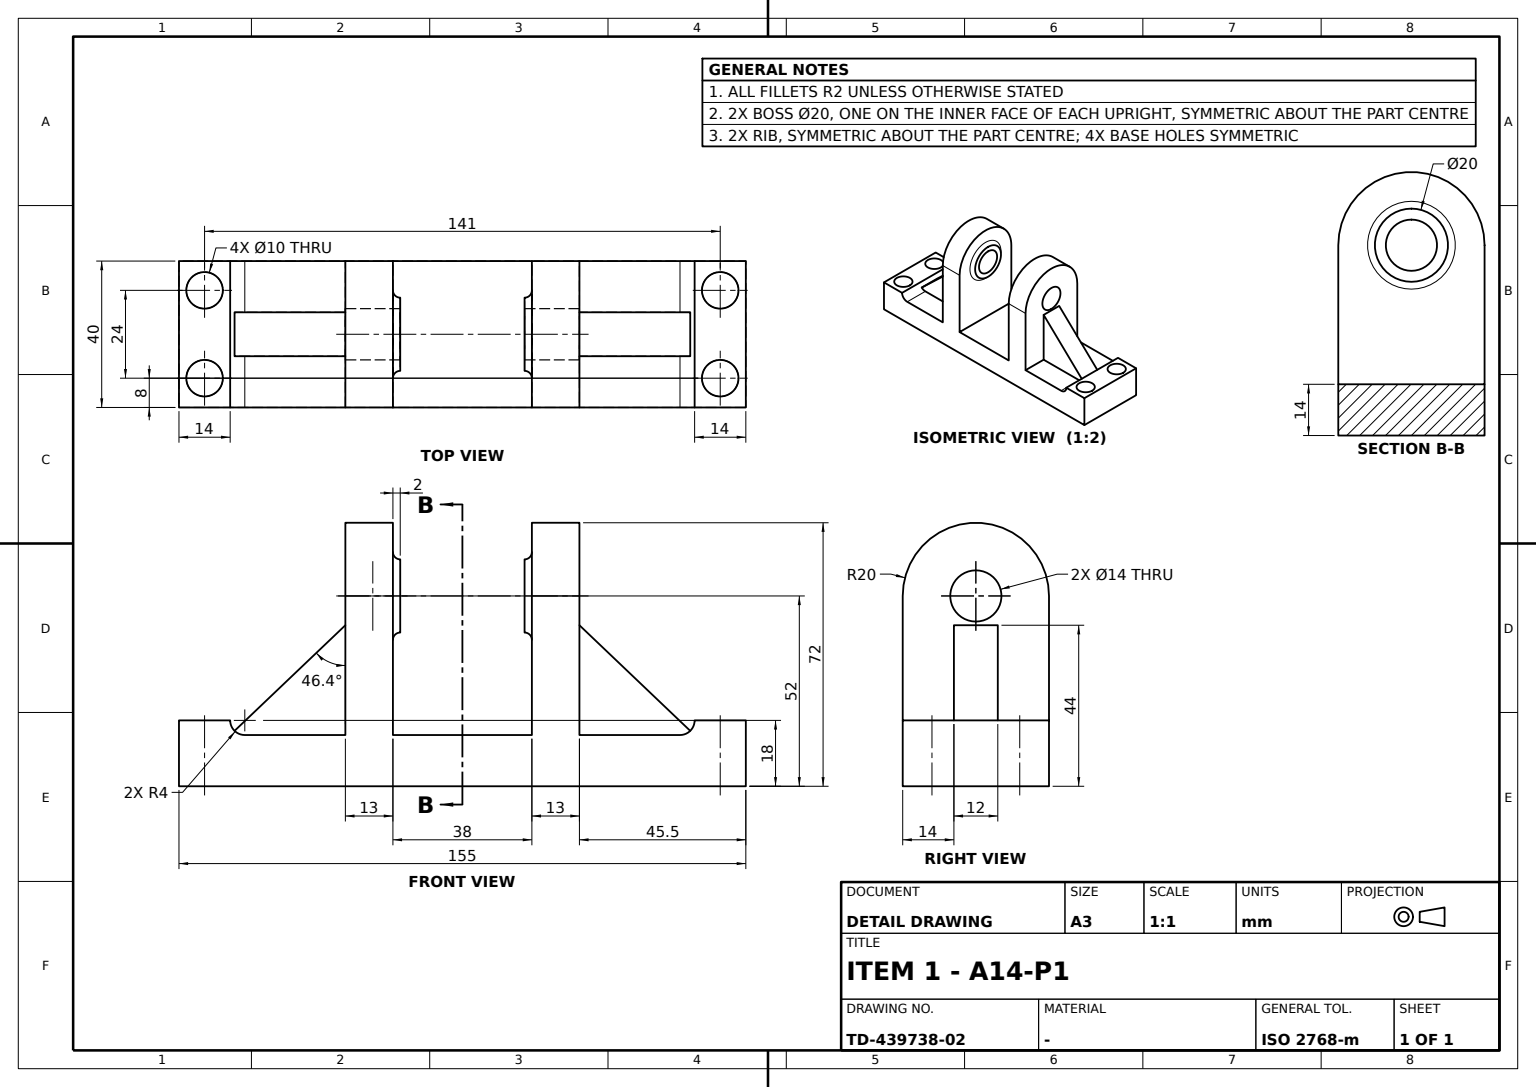
ISO-10303-21;
HEADER;
FILE_DESCRIPTION((''),'2;1');
FILE_NAME('','',(''),(''),'','','');
FILE_SCHEMA(('AUTOMOTIVE_DESIGN'));
ENDSEC;
DATA;
#1=APPLICATION_CONTEXT('');
#2=PRODUCT_CONTEXT('',#1,'mechanical');
#3=PRODUCT('','','',(#2));
#4=PRODUCT_DEFINITION_FORMATION('','',#3);
#5=PRODUCT_DEFINITION_CONTEXT('',#1,'design');
#6=PRODUCT_DEFINITION('','',#4,#5);
#7=PRODUCT_DEFINITION_SHAPE('','',#6);
#8=(LENGTH_UNIT()NAMED_UNIT(*)SI_UNIT(.MILLI.,.METRE.));
#9=(NAMED_UNIT(*)PLANE_ANGLE_UNIT()SI_UNIT($,.RADIAN.));
#10=(NAMED_UNIT(*)SI_UNIT($,.STERADIAN.)SOLID_ANGLE_UNIT());
#11=UNCERTAINTY_MEASURE_WITH_UNIT(LENGTH_MEASURE(0.005),#8,'distance_accuracy_value','');
#12=(GEOMETRIC_REPRESENTATION_CONTEXT(3)GLOBAL_UNCERTAINTY_ASSIGNED_CONTEXT((#11))GLOBAL_UNIT_ASSIGNED_CONTEXT((#8,#9,#10))REPRESENTATION_CONTEXT('',''));
#13=CARTESIAN_POINT('',(17.,0.,42.));
#14=VERTEX_POINT('',#13);
#15=CARTESIAN_POINT('',(17.,0.,52.));
#16=DIRECTION('',(1.,0.,0.));
#17=DIRECTION('',(0.,0.,-1.));
#18=AXIS2_PLACEMENT_3D('',#15,#16,#17);
#19=CIRCLE('',#18,10.);
#20=EDGE_CURVE('',#14,#14,#19,.T.);
#21=ORIENTED_EDGE('',*,*,#20,.F.);
#22=EDGE_LOOP('',(#21));
#23=FACE_BOUND('',#22,.T.);
#24=CARTESIAN_POINT('',(17.,0.,45.));
#25=VERTEX_POINT('',#24);
#26=CIRCLE('',#18,7.);
#27=EDGE_CURVE('',#25,#25,#26,.T.);
#28=ORIENTED_EDGE('',*,*,#27,.T.);
#29=EDGE_LOOP('',(#28));
#30=FACE_BOUND('',#29,.T.);
#31=CARTESIAN_POINT('',(17.,0.,14.));
#32=DIRECTION('',(0.,0.,1.));
#33=AXIS2_PLACEMENT_3D('',#31,#16,#32);
#34=PLANE('',#33);
#35=ADVANCED_FACE('',(#23,#30),#34,.F.);
#36=CARTESIAN_POINT('',(-75.5,12.,0.));
#37=VERTEX_POINT('',#36);
#38=CARTESIAN_POINT('',(-70.5,12.,0.));
#39=DIRECTION('',(-1.,0.,0.));
#40=AXIS2_PLACEMENT_3D('',#38,#17,#39);
#41=CIRCLE('',#40,5.);
#42=EDGE_CURVE('',#37,#37,#41,.T.);
#43=ORIENTED_EDGE('',*,*,#42,.T.);
#44=EDGE_LOOP('',(#43));
#45=FACE_BOUND('',#44,.T.);
#46=CARTESIAN_POINT('',(-65.5,12.,18.));
#47=VERTEX_POINT('',#46);
#48=CARTESIAN_POINT('',(-70.5,12.,18.));
#49=AXIS2_PLACEMENT_3D('',#48,#32,#16);
#50=CIRCLE('',#49,5.);
#51=EDGE_CURVE('',#47,#47,#50,.T.);
#52=ORIENTED_EDGE('',*,*,#51,.T.);
#53=EDGE_LOOP('',(#52));
#54=FACE_BOUND('',#53,.T.);
#55=CARTESIAN_POINT('',(-70.5,12.,-18.5));
#56=DIRECTION('',(0.,1.,0.));
#57=AXIS2_PLACEMENT_3D('',#55,#32,#56);
#58=CYLINDRICAL_SURFACE('',#57,5.);
#59=ADVANCED_FACE('',(#45,#54),#58,.F.);
#60=CARTESIAN_POINT('',(75.5,-12.,18.));
#61=VERTEX_POINT('',#60);
#62=CARTESIAN_POINT('',(70.5,-12.,18.));
#63=AXIS2_PLACEMENT_3D('',#62,#32,#16);
#64=CIRCLE('',#63,5.);
#65=EDGE_CURVE('',#61,#61,#64,.T.);
#66=ORIENTED_EDGE('',*,*,#65,.T.);
#67=EDGE_LOOP('',(#66));
#68=FACE_BOUND('',#67,.T.);
#69=CARTESIAN_POINT('',(65.5,-12.,0.));
#70=VERTEX_POINT('',#69);
#71=CARTESIAN_POINT('',(70.5,-12.,0.));
#72=AXIS2_PLACEMENT_3D('',#71,#17,#39);
#73=CIRCLE('',#72,5.);
#74=EDGE_CURVE('',#70,#70,#73,.T.);
#75=ORIENTED_EDGE('',*,*,#74,.T.);
#76=EDGE_LOOP('',(#75));
#77=FACE_BOUND('',#76,.T.);
#78=CARTESIAN_POINT('',(70.5,-12.,-18.5));
#79=AXIS2_PLACEMENT_3D('',#78,#32,#56);
#80=CYLINDRICAL_SURFACE('',#79,5.);
#81=ADVANCED_FACE('',(#68,#77),#80,.F.);
#82=ORIENTED_EDGE('',*,*,#27,.F.);
#83=EDGE_LOOP('',(#82));
#84=FACE_BOUND('',#83,.T.);
#85=CARTESIAN_POINT('',(32.,0.,45.));
#86=VERTEX_POINT('',#85);
#87=CARTESIAN_POINT('',(32.,0.,52.));
#88=AXIS2_PLACEMENT_3D('',#87,#16,#17);
#89=CIRCLE('',#88,7.);
#90=EDGE_CURVE('',#86,#86,#89,.T.);
#91=ORIENTED_EDGE('',*,*,#90,.T.);
#92=EDGE_LOOP('',(#91));
#93=FACE_BOUND('',#92,.T.);
#94=CARTESIAN_POINT('',(4.5,0.,52.));
#95=DIRECTION('',(0.,-1.,0.));
#96=AXIS2_PLACEMENT_3D('',#94,#39,#95);
#97=CYLINDRICAL_SURFACE('',#96,7.);
#98=ADVANCED_FACE('',(#84,#93),#97,.F.);
#99=ORIENTED_EDGE('',*,*,#90,.F.);
#100=EDGE_LOOP('',(#99));
#101=FACE_BOUND('',#100,.T.);
#102=CARTESIAN_POINT('',(32.,6.,44.));
#103=VERTEX_POINT('',#102);
#104=CARTESIAN_POINT('',(32.,6.,14.));
#105=VERTEX_POINT('',#104);
#106=CARTESIAN_POINT('',(32.,6.,0.));
#107=VECTOR('',#17,1000.);
#108=LINE('',#106,#107);
#109=EDGE_CURVE('',#103,#105,#108,.T.);
#110=ORIENTED_EDGE('',*,*,#109,.T.);
#111=CARTESIAN_POINT('',(32.,20.,14.));
#112=VERTEX_POINT('',#111);
#113=CARTESIAN_POINT('',(32.,0.,14.));
#114=VECTOR('',#56,1000.);
#115=LINE('',#113,#114);
#116=EDGE_CURVE('',#105,#112,#115,.T.);
#117=ORIENTED_EDGE('',*,*,#116,.T.);
#118=CARTESIAN_POINT('',(32.,20.,52.));
#119=VERTEX_POINT('',#118);
#120=CARTESIAN_POINT('',(32.,20.,0.));
#121=VECTOR('',#32,1000.);
#122=LINE('',#120,#121);
#123=EDGE_CURVE('',#112,#119,#122,.T.);
#124=ORIENTED_EDGE('',*,*,#123,.T.);
#125=CARTESIAN_POINT('',(32.,-20.,52.));
#126=VERTEX_POINT('',#125);
#127=CIRCLE('',#88,20.);
#128=EDGE_CURVE('',#119,#126,#127,.T.);
#129=ORIENTED_EDGE('',*,*,#128,.T.);
#130=CARTESIAN_POINT('',(32.,-20.,14.));
#131=VERTEX_POINT('',#130);
#132=CARTESIAN_POINT('',(32.,-20.,0.));
#133=LINE('',#132,#107);
#134=EDGE_CURVE('',#126,#131,#133,.T.);
#135=ORIENTED_EDGE('',*,*,#134,.T.);
#136=CARTESIAN_POINT('',(32.,-6.,14.));
#137=VERTEX_POINT('',#136);
#138=EDGE_CURVE('',#131,#137,#115,.T.);
#139=ORIENTED_EDGE('',*,*,#138,.T.);
#140=CARTESIAN_POINT('',(32.,-6.,44.));
#141=VERTEX_POINT('',#140);
#142=CARTESIAN_POINT('',(32.,-6.,0.));
#143=LINE('',#142,#107);
#144=EDGE_CURVE('',#141,#137,#143,.T.);
#145=ORIENTED_EDGE('',*,*,#144,.F.);
#146=CARTESIAN_POINT('',(32.,0.,44.));
#147=LINE('',#146,#114);
#148=EDGE_CURVE('',#141,#103,#147,.T.);
#149=ORIENTED_EDGE('',*,*,#148,.T.);
#150=EDGE_LOOP('',(#110,#117,#124,#129,#135,#139,#145,#149));
#151=FACE_BOUND('',#150,.T.);
#152=CARTESIAN_POINT('',(32.,0.,0.));
#153=AXIS2_PLACEMENT_3D('',#152,#16,#56);
#154=PLANE('',#153);
#155=ADVANCED_FACE('',(#101,#151),#154,.T.);
#156=ORIENTED_EDGE('',*,*,#128,.F.);
#157=CARTESIAN_POINT('',(19.,20.,52.));
#158=VERTEX_POINT('',#157);
#159=CARTESIAN_POINT('',(0.,20.,52.));
#160=VECTOR('',#16,1000.);
#161=LINE('',#159,#160);
#162=EDGE_CURVE('',#158,#119,#161,.T.);
#163=ORIENTED_EDGE('',*,*,#162,.F.);
#164=CARTESIAN_POINT('',(19.,-20.,52.));
#165=VERTEX_POINT('',#164);
#166=CARTESIAN_POINT('',(19.,0.,52.));
#167=AXIS2_PLACEMENT_3D('',#166,#16,#17);
#168=CIRCLE('',#167,20.);
#169=EDGE_CURVE('',#158,#165,#168,.T.);
#170=ORIENTED_EDGE('',*,*,#169,.T.);
#171=CARTESIAN_POINT('',(0.,-20.,52.));
#172=LINE('',#171,#160);
#173=EDGE_CURVE('',#165,#126,#172,.T.);
#174=ORIENTED_EDGE('',*,*,#173,.T.);
#175=EDGE_LOOP('',(#156,#163,#170,#174));
#176=FACE_BOUND('',#175,.T.);
#177=CARTESIAN_POINT('',(0.,0.,52.));
#178=AXIS2_PLACEMENT_3D('',#177,#16,#56);
#179=CYLINDRICAL_SURFACE('',#178,20.);
#180=ADVANCED_FACE('',(#176),#179,.T.);
#181=CARTESIAN_POINT('',(-59.5,20.,14.));
#182=VERTEX_POINT('',#181);
#183=CARTESIAN_POINT('',(-63.5,20.,18.));
#184=VERTEX_POINT('',#183);
#185=CARTESIAN_POINT('',(-59.5,20.,18.));
#186=AXIS2_PLACEMENT_3D('',#185,#56,#32);
#187=CIRCLE('',#186,4.);
#188=EDGE_CURVE('',#182,#184,#187,.T.);
#189=ORIENTED_EDGE('',*,*,#188,.T.);
#190=CARTESIAN_POINT('',(-63.5,-20.,18.));
#191=VERTEX_POINT('',#190);
#192=LINE('',#190,#114);
#193=EDGE_CURVE('',#191,#184,#192,.T.);
#194=ORIENTED_EDGE('',*,*,#193,.F.);
#195=CARTESIAN_POINT('',(-59.5,-20.,14.));
#196=VERTEX_POINT('',#195);
#197=CARTESIAN_POINT('',(-59.5,-20.,18.));
#198=AXIS2_PLACEMENT_3D('',#197,#95,#17);
#199=CIRCLE('',#198,4.);
#200=EDGE_CURVE('',#191,#196,#199,.T.);
#201=ORIENTED_EDGE('',*,*,#200,.T.);
#202=CARTESIAN_POINT('',(-59.5,-6.,14.));
#203=VERTEX_POINT('',#202);
#204=CARTESIAN_POINT('',(-59.5,0.,14.));
#205=LINE('',#204,#114);
#206=EDGE_CURVE('',#196,#203,#205,.T.);
#207=ORIENTED_EDGE('',*,*,#206,.T.);
#208=CARTESIAN_POINT('',(-62.299704,-6.,15.143139));
#209=VERTEX_POINT('',#208);
#210=CARTESIAN_POINT('',(-59.5,-6.,18.));
#211=AXIS2_PLACEMENT_3D('',#210,#56,#32);
#212=CIRCLE('',#211,4.);
#213=EDGE_CURVE('',#203,#209,#212,.T.);
#214=ORIENTED_EDGE('',*,*,#213,.T.);
#215=CARTESIAN_POINT('',(-62.299704,6.,15.143139));
#216=VERTEX_POINT('',#215);
#217=LINE('',#215,#114);
#218=EDGE_CURVE('',#216,#209,#217,.F.);
#219=ORIENTED_EDGE('',*,*,#218,.F.);
#220=CARTESIAN_POINT('',(-59.5,6.,14.));
#221=VERTEX_POINT('',#220);
#222=CARTESIAN_POINT('',(-59.5,6.,18.));
#223=AXIS2_PLACEMENT_3D('',#222,#56,#32);
#224=CIRCLE('',#223,4.);
#225=EDGE_CURVE('',#221,#216,#224,.T.);
#226=ORIENTED_EDGE('',*,*,#225,.F.);
#227=EDGE_CURVE('',#221,#182,#205,.T.);
#228=ORIENTED_EDGE('',*,*,#227,.T.);
#229=EDGE_LOOP('',(#189,#194,#201,#207,#214,#219,#226,#228));
#230=FACE_BOUND('',#229,.T.);
#231=CARTESIAN_POINT('',(-59.5,0.,18.));
#232=AXIS2_PLACEMENT_3D('',#231,#56,#17);
#233=CYLINDRICAL_SURFACE('',#232,4.);
#234=ADVANCED_FACE('',(#230),#233,.F.);
#235=CARTESIAN_POINT('',(-32.,-20.,14.));
#236=VERTEX_POINT('',#235);
#237=CARTESIAN_POINT('',(-32.,-6.,14.));
#238=VERTEX_POINT('',#237);
#239=CARTESIAN_POINT('',(-32.,0.,14.));
#240=LINE('',#239,#114);
#241=EDGE_CURVE('',#236,#238,#240,.T.);
#242=ORIENTED_EDGE('',*,*,#241,.T.);
#243=CARTESIAN_POINT('',(0.,-6.,14.));
#244=LINE('',#243,#160);
#245=EDGE_CURVE('',#203,#238,#244,.T.);
#246=ORIENTED_EDGE('',*,*,#245,.F.);
#247=ORIENTED_EDGE('',*,*,#206,.F.);
#248=CARTESIAN_POINT('',(-63.5,-20.,14.));
#249=LINE('',#248,#160);
#250=EDGE_CURVE('',#196,#236,#249,.T.);
#251=ORIENTED_EDGE('',*,*,#250,.T.);
#252=EDGE_LOOP('',(#242,#246,#247,#251));
#253=FACE_BOUND('',#252,.T.);
#254=CARTESIAN_POINT('',(-63.5,0.,14.));
#255=AXIS2_PLACEMENT_3D('',#254,#32,#16);
#256=PLANE('',#255);
#257=ADVANCED_FACE('',(#253),#256,.T.);
#258=CARTESIAN_POINT('',(19.,-20.,14.));
#259=VERTEX_POINT('',#258);
#260=CARTESIAN_POINT('',(19.,20.,14.));
#261=VERTEX_POINT('',#260);
#262=CARTESIAN_POINT('',(19.,0.,14.));
#263=LINE('',#262,#114);
#264=EDGE_CURVE('',#259,#261,#263,.T.);
#265=ORIENTED_EDGE('',*,*,#264,.T.);
#266=CARTESIAN_POINT('',(-19.,20.,14.));
#267=VERTEX_POINT('',#266);
#268=CARTESIAN_POINT('',(0.,20.,14.));
#269=LINE('',#268,#160);
#270=EDGE_CURVE('',#267,#261,#269,.T.);
#271=ORIENTED_EDGE('',*,*,#270,.F.);
#272=CARTESIAN_POINT('',(-19.,-20.,14.));
#273=VERTEX_POINT('',#272);
#274=LINE('',#266,#114);
#275=EDGE_CURVE('',#273,#267,#274,.T.);
#276=ORIENTED_EDGE('',*,*,#275,.F.);
#277=EDGE_CURVE('',#273,#259,#249,.T.);
#278=ORIENTED_EDGE('',*,*,#277,.T.);
#279=EDGE_LOOP('',(#265,#271,#276,#278));
#280=FACE_BOUND('',#279,.T.);
#281=ADVANCED_FACE('',(#280),#256,.T.);
#282=CARTESIAN_POINT('',(75.5,12.,18.));
#283=VERTEX_POINT('',#282);
#284=CARTESIAN_POINT('',(70.5,12.,18.));
#285=AXIS2_PLACEMENT_3D('',#284,#32,#16);
#286=CIRCLE('',#285,5.);
#287=EDGE_CURVE('',#283,#283,#286,.T.);
#288=ORIENTED_EDGE('',*,*,#287,.T.);
#289=EDGE_LOOP('',(#288));
#290=FACE_BOUND('',#289,.T.);
#291=CARTESIAN_POINT('',(65.5,12.,0.));
#292=VERTEX_POINT('',#291);
#293=CARTESIAN_POINT('',(70.5,12.,0.));
#294=AXIS2_PLACEMENT_3D('',#293,#17,#39);
#295=CIRCLE('',#294,5.);
#296=EDGE_CURVE('',#292,#292,#295,.T.);
#297=ORIENTED_EDGE('',*,*,#296,.T.);
#298=EDGE_LOOP('',(#297));
#299=FACE_BOUND('',#298,.T.);
#300=CARTESIAN_POINT('',(70.5,12.,-18.5));
#301=AXIS2_PLACEMENT_3D('',#300,#32,#56);
#302=CYLINDRICAL_SURFACE('',#301,5.);
#303=ADVANCED_FACE('',(#290,#299),#302,.F.);
#304=CARTESIAN_POINT('',(77.5,-20.,0.));
#305=VERTEX_POINT('',#304);
#306=CARTESIAN_POINT('',(77.5,20.,0.));
#307=VERTEX_POINT('',#306);
#308=CARTESIAN_POINT('',(77.5,0.,0.));
#309=LINE('',#308,#114);
#310=EDGE_CURVE('',#305,#307,#309,.T.);
#311=ORIENTED_EDGE('',*,*,#310,.T.);
#312=CARTESIAN_POINT('',(77.5,20.,18.));
#313=VERTEX_POINT('',#312);
#314=LINE('',#306,#107);
#315=EDGE_CURVE('',#313,#307,#314,.T.);
#316=ORIENTED_EDGE('',*,*,#315,.F.);
#317=CARTESIAN_POINT('',(77.5,-20.,18.));
#318=VERTEX_POINT('',#317);
#319=CARTESIAN_POINT('',(77.5,0.,18.));
#320=LINE('',#319,#114);
#321=EDGE_CURVE('',#318,#313,#320,.T.);
#322=ORIENTED_EDGE('',*,*,#321,.F.);
#323=LINE('',#317,#107);
#324=EDGE_CURVE('',#318,#305,#323,.T.);
#325=ORIENTED_EDGE('',*,*,#324,.T.);
#326=EDGE_LOOP('',(#311,#316,#322,#325));
#327=FACE_BOUND('',#326,.T.);
#328=AXIS2_PLACEMENT_3D('',#319,#16,#17);
#329=PLANE('',#328);
#330=ADVANCED_FACE('',(#327),#329,.T.);
#331=CARTESIAN_POINT('',(-77.5,-20.,18.));
#332=VERTEX_POINT('',#331);
#333=LINE('',#331,#160);
#334=EDGE_CURVE('',#332,#191,#333,.T.);
#335=ORIENTED_EDGE('',*,*,#334,.F.);
#336=CARTESIAN_POINT('',(-77.5,-20.,0.));
#337=VERTEX_POINT('',#336);
#338=LINE('',#336,#121);
#339=EDGE_CURVE('',#337,#332,#338,.T.);
#340=ORIENTED_EDGE('',*,*,#339,.F.);
#341=CARTESIAN_POINT('',(0.,-20.,0.));
#342=VECTOR('',#39,1000.);
#343=LINE('',#341,#342);
#344=EDGE_CURVE('',#305,#337,#343,.T.);
#345=ORIENTED_EDGE('',*,*,#344,.F.);
#346=ORIENTED_EDGE('',*,*,#324,.F.);
#347=CARTESIAN_POINT('',(63.5,-20.,18.));
#348=VERTEX_POINT('',#347);
#349=EDGE_CURVE('',#348,#318,#333,.T.);
#350=ORIENTED_EDGE('',*,*,#349,.F.);
#351=CARTESIAN_POINT('',(59.5,-20.,14.));
#352=VERTEX_POINT('',#351);
#353=CARTESIAN_POINT('',(59.5,-20.,18.));
#354=AXIS2_PLACEMENT_3D('',#353,#95,#17);
#355=CIRCLE('',#354,4.);
#356=EDGE_CURVE('',#352,#348,#355,.T.);
#357=ORIENTED_EDGE('',*,*,#356,.F.);
#358=EDGE_CURVE('',#131,#352,#249,.T.);
#359=ORIENTED_EDGE('',*,*,#358,.F.);
#360=ORIENTED_EDGE('',*,*,#134,.F.);
#361=ORIENTED_EDGE('',*,*,#173,.F.);
#362=CARTESIAN_POINT('',(19.,-20.,-6.034836));
#363=LINE('',#362,#107);
#364=EDGE_CURVE('',#165,#259,#363,.T.);
#365=ORIENTED_EDGE('',*,*,#364,.T.);
#366=ORIENTED_EDGE('',*,*,#277,.F.);
#367=CARTESIAN_POINT('',(-19.,-20.,52.));
#368=VERTEX_POINT('',#367);
#369=LINE('',#367,#107);
#370=EDGE_CURVE('',#368,#273,#369,.T.);
#371=ORIENTED_EDGE('',*,*,#370,.F.);
#372=CARTESIAN_POINT('',(-32.,-20.,52.));
#373=VERTEX_POINT('',#372);
#374=EDGE_CURVE('',#373,#368,#172,.T.);
#375=ORIENTED_EDGE('',*,*,#374,.F.);
#376=CARTESIAN_POINT('',(-32.,-20.,0.));
#377=LINE('',#376,#107);
#378=EDGE_CURVE('',#373,#236,#377,.T.);
#379=ORIENTED_EDGE('',*,*,#378,.T.);
#380=ORIENTED_EDGE('',*,*,#250,.F.);
#381=ORIENTED_EDGE('',*,*,#200,.F.);
#382=EDGE_LOOP('',(#335,#340,#345,#346,#350,#357,#359,#360,#361,#365,#366,#371,#375,#379,#380,#381));
#383=FACE_BOUND('',#382,.T.);
#384=AXIS2_PLACEMENT_3D('',#171,#95,#17);
#385=PLANE('',#384);
#386=ADVANCED_FACE('',(#383),#385,.T.);
#387=CARTESIAN_POINT('',(-17.,0.,62.));
#388=VERTEX_POINT('',#387);
#389=CARTESIAN_POINT('',(-17.,0.,52.));
#390=AXIS2_PLACEMENT_3D('',#389,#39,#32);
#391=CIRCLE('',#390,10.);
#392=EDGE_CURVE('',#388,#388,#391,.T.);
#393=ORIENTED_EDGE('',*,*,#392,.F.);
#394=EDGE_LOOP('',(#393));
#395=FACE_BOUND('',#394,.T.);
#396=CARTESIAN_POINT('',(-17.,0.,59.));
#397=VERTEX_POINT('',#396);
#398=CIRCLE('',#390,7.);
#399=EDGE_CURVE('',#397,#397,#398,.T.);
#400=ORIENTED_EDGE('',*,*,#399,.T.);
#401=EDGE_LOOP('',(#400));
#402=FACE_BOUND('',#401,.T.);
#403=CARTESIAN_POINT('',(-17.,0.,85.919682));
#404=AXIS2_PLACEMENT_3D('',#403,#39,#17);
#405=PLANE('',#404);
#406=ADVANCED_FACE('',(#395,#402),#405,.F.);
#407=CARTESIAN_POINT('',(-32.,20.,14.));
#408=VERTEX_POINT('',#407);
#409=EDGE_CURVE('',#182,#408,#269,.T.);
#410=ORIENTED_EDGE('',*,*,#409,.F.);
#411=ORIENTED_EDGE('',*,*,#227,.F.);
#412=CARTESIAN_POINT('',(-32.,6.,14.));
#413=VERTEX_POINT('',#412);
#414=CARTESIAN_POINT('',(0.,6.,14.));
#415=LINE('',#414,#160);
#416=EDGE_CURVE('',#221,#413,#415,.T.);
#417=ORIENTED_EDGE('',*,*,#416,.T.);
#418=EDGE_CURVE('',#413,#408,#240,.T.);
#419=ORIENTED_EDGE('',*,*,#418,.T.);
#420=EDGE_LOOP('',(#410,#411,#417,#419));
#421=FACE_BOUND('',#420,.T.);
#422=ADVANCED_FACE('',(#421),#256,.T.);
#423=CARTESIAN_POINT('',(-32.,6.,44.));
#424=VERTEX_POINT('',#423);
#425=CARTESIAN_POINT('',(-37.193817,6.,39.053508));
#426=DIRECTION('',(0.724137931,0.,0.689655172));
#427=VECTOR('',#426,1000.);
#428=LINE('',#425,#427);
#429=EDGE_CURVE('',#216,#424,#428,.T.);
#430=ORIENTED_EDGE('',*,*,#429,.F.);
#431=ORIENTED_EDGE('',*,*,#218,.T.);
#432=CARTESIAN_POINT('',(-32.,-6.,44.));
#433=VERTEX_POINT('',#432);
#434=CARTESIAN_POINT('',(-37.193817,-6.,39.053508));
#435=LINE('',#434,#427);
#436=EDGE_CURVE('',#209,#433,#435,.T.);
#437=ORIENTED_EDGE('',*,*,#436,.T.);
#438=CARTESIAN_POINT('',(-32.,0.,44.));
#439=LINE('',#438,#114);
#440=EDGE_CURVE('',#433,#424,#439,.T.);
#441=ORIENTED_EDGE('',*,*,#440,.T.);
#442=EDGE_LOOP('',(#430,#431,#437,#441));
#443=FACE_BOUND('',#442,.T.);
#444=DIRECTION('',(-0.689655172,0.,0.724137931));
#445=AXIS2_PLACEMENT_3D('',#254,#444,#426);
#446=PLANE('',#445);
#447=ADVANCED_FACE('',(#443),#446,.T.);
#448=CARTESIAN_POINT('',(19.,0.,40.));
#449=VERTEX_POINT('',#448);
#450=CIRCLE('',#167,12.);
#451=EDGE_CURVE('',#449,#449,#450,.T.);
#452=ORIENTED_EDGE('',*,*,#451,.F.);
#453=EDGE_LOOP('',(#452));
#454=FACE_BOUND('',#453,.T.);
#455=ORIENTED_EDGE('',*,*,#20,.T.);
#456=EDGE_LOOP('',(#455));
#457=FACE_BOUND('',#456,.T.);
#458=DIRECTION('',(0.,-0.5,0.866025404));
#459=AXIS2_PLACEMENT_3D('',#15,#16,#458);
#460=TOROIDAL_SURFACE('',#459,12.,2.);
#461=ADVANCED_FACE('',(#454,#457),#460,.F.);
#462=CARTESIAN_POINT('',(-32.,-6.,0.));
#463=LINE('',#462,#107);
#464=EDGE_CURVE('',#433,#238,#463,.T.);
#465=ORIENTED_EDGE('',*,*,#464,.F.);
#466=ORIENTED_EDGE('',*,*,#436,.F.);
#467=ORIENTED_EDGE('',*,*,#213,.F.);
#468=ORIENTED_EDGE('',*,*,#245,.T.);
#469=EDGE_LOOP('',(#465,#466,#467,#468));
#470=FACE_BOUND('',#469,.T.);
#471=CARTESIAN_POINT('',(0.,-6.,0.));
#472=AXIS2_PLACEMENT_3D('',#471,#56,#39);
#473=PLANE('',#472);
#474=ADVANCED_FACE('',(#470),#473,.F.);
#475=CARTESIAN_POINT('',(-32.,20.,52.));
#476=VERTEX_POINT('',#475);
#477=CARTESIAN_POINT('',(-19.,20.,52.));
#478=VERTEX_POINT('',#477);
#479=EDGE_CURVE('',#476,#478,#161,.T.);
#480=ORIENTED_EDGE('',*,*,#479,.T.);
#481=CARTESIAN_POINT('',(-19.,20.,83.965164));
#482=LINE('',#481,#107);
#483=EDGE_CURVE('',#478,#267,#482,.T.);
#484=ORIENTED_EDGE('',*,*,#483,.T.);
#485=ORIENTED_EDGE('',*,*,#270,.T.);
#486=CARTESIAN_POINT('',(19.,20.,-6.034836));
#487=LINE('',#486,#121);
#488=EDGE_CURVE('',#261,#158,#487,.T.);
#489=ORIENTED_EDGE('',*,*,#488,.T.);
#490=ORIENTED_EDGE('',*,*,#162,.T.);
#491=ORIENTED_EDGE('',*,*,#123,.F.);
#492=CARTESIAN_POINT('',(59.5,20.,14.));
#493=VERTEX_POINT('',#492);
#494=EDGE_CURVE('',#112,#493,#269,.T.);
#495=ORIENTED_EDGE('',*,*,#494,.T.);
#496=CARTESIAN_POINT('',(63.5,20.,18.));
#497=VERTEX_POINT('',#496);
#498=CARTESIAN_POINT('',(59.5,20.,18.));
#499=AXIS2_PLACEMENT_3D('',#498,#56,#32);
#500=CIRCLE('',#499,4.);
#501=EDGE_CURVE('',#497,#493,#500,.T.);
#502=ORIENTED_EDGE('',*,*,#501,.F.);
#503=CARTESIAN_POINT('',(0.,20.,18.));
#504=LINE('',#503,#160);
#505=EDGE_CURVE('',#497,#313,#504,.T.);
#506=ORIENTED_EDGE('',*,*,#505,.T.);
#507=ORIENTED_EDGE('',*,*,#315,.T.);
#508=CARTESIAN_POINT('',(-77.5,20.,0.));
#509=VERTEX_POINT('',#508);
#510=CARTESIAN_POINT('',(0.,20.,0.));
#511=LINE('',#510,#342);
#512=EDGE_CURVE('',#307,#509,#511,.T.);
#513=ORIENTED_EDGE('',*,*,#512,.T.);
#514=CARTESIAN_POINT('',(-77.5,20.,18.));
#515=VERTEX_POINT('',#514);
#516=LINE('',#508,#121);
#517=EDGE_CURVE('',#509,#515,#516,.T.);
#518=ORIENTED_EDGE('',*,*,#517,.T.);
#519=EDGE_CURVE('',#515,#184,#504,.T.);
#520=ORIENTED_EDGE('',*,*,#519,.T.);
#521=ORIENTED_EDGE('',*,*,#188,.F.);
#522=ORIENTED_EDGE('',*,*,#409,.T.);
#523=CARTESIAN_POINT('',(-32.,20.,0.));
#524=LINE('',#523,#121);
#525=EDGE_CURVE('',#408,#476,#524,.T.);
#526=ORIENTED_EDGE('',*,*,#525,.T.);
#527=EDGE_LOOP('',(#480,#484,#485,#489,#490,#491,#495,#502,#506,#507,#513,#518,#520,#521,#522,#526));
#528=FACE_BOUND('',#527,.T.);
#529=AXIS2_PLACEMENT_3D('',#510,#56,#32);
#530=PLANE('',#529);
#531=ADVANCED_FACE('',(#528),#530,.T.);
#532=ORIENTED_EDGE('',*,*,#65,.F.);
#533=EDGE_LOOP('',(#532));
#534=FACE_BOUND('',#533,.T.);
#535=CARTESIAN_POINT('',(63.5,-6.,18.));
#536=LINE('',#535,#114);
#537=EDGE_CURVE('',#348,#497,#536,.T.);
#538=ORIENTED_EDGE('',*,*,#537,.F.);
#539=ORIENTED_EDGE('',*,*,#349,.T.);
#540=ORIENTED_EDGE('',*,*,#321,.T.);
#541=ORIENTED_EDGE('',*,*,#505,.F.);
#542=EDGE_LOOP('',(#538,#539,#540,#541));
#543=FACE_BOUND('',#542,.T.);
#544=ORIENTED_EDGE('',*,*,#287,.F.);
#545=EDGE_LOOP('',(#544));
#546=FACE_BOUND('',#545,.T.);
#547=CARTESIAN_POINT('',(-77.5,0.,18.));
#548=AXIS2_PLACEMENT_3D('',#547,#32,#16);
#549=PLANE('',#548);
#550=ADVANCED_FACE('',(#534,#543,#546),#549,.T.);
#551=ORIENTED_EDGE('',*,*,#193,.T.);
#552=ORIENTED_EDGE('',*,*,#519,.F.);
#553=LINE('',#547,#114);
#554=EDGE_CURVE('',#332,#515,#553,.T.);
#555=ORIENTED_EDGE('',*,*,#554,.F.);
#556=ORIENTED_EDGE('',*,*,#334,.T.);
#557=EDGE_LOOP('',(#551,#552,#555,#556));
#558=FACE_BOUND('',#557,.T.);
#559=CARTESIAN_POINT('',(-65.5,-12.,18.));
#560=VERTEX_POINT('',#559);
#561=CARTESIAN_POINT('',(-70.5,-12.,18.));
#562=AXIS2_PLACEMENT_3D('',#561,#32,#16);
#563=CIRCLE('',#562,5.);
#564=EDGE_CURVE('',#560,#560,#563,.T.);
#565=ORIENTED_EDGE('',*,*,#564,.F.);
#566=EDGE_LOOP('',(#565));
#567=FACE_BOUND('',#566,.T.);
#568=ORIENTED_EDGE('',*,*,#51,.F.);
#569=EDGE_LOOP('',(#568));
#570=FACE_BOUND('',#569,.T.);
#571=ADVANCED_FACE('',(#558,#567,#570),#549,.T.);
#572=ORIENTED_EDGE('',*,*,#494,.F.);
#573=ORIENTED_EDGE('',*,*,#116,.F.);
#574=CARTESIAN_POINT('',(59.5,6.,14.));
#575=VERTEX_POINT('',#574);
#576=EDGE_CURVE('',#105,#575,#415,.T.);
#577=ORIENTED_EDGE('',*,*,#576,.T.);
#578=CARTESIAN_POINT('',(59.5,0.,14.));
#579=LINE('',#578,#114);
#580=EDGE_CURVE('',#575,#493,#579,.T.);
#581=ORIENTED_EDGE('',*,*,#580,.T.);
#582=EDGE_LOOP('',(#572,#573,#577,#581));
#583=FACE_BOUND('',#582,.T.);
#584=ADVANCED_FACE('',(#583),#256,.T.);
#585=ORIENTED_EDGE('',*,*,#399,.F.);
#586=EDGE_LOOP('',(#585));
#587=FACE_BOUND('',#586,.T.);
#588=CARTESIAN_POINT('',(-32.,0.,45.));
#589=VERTEX_POINT('',#588);
#590=CARTESIAN_POINT('',(-32.,0.,52.));
#591=AXIS2_PLACEMENT_3D('',#590,#16,#17);
#592=CIRCLE('',#591,7.);
#593=EDGE_CURVE('',#589,#589,#592,.F.);
#594=ORIENTED_EDGE('',*,*,#593,.T.);
#595=EDGE_LOOP('',(#594));
#596=FACE_BOUND('',#595,.T.);
#597=ADVANCED_FACE('',(#587,#596),#97,.F.);
#598=ORIENTED_EDGE('',*,*,#564,.T.);
#599=EDGE_LOOP('',(#598));
#600=FACE_BOUND('',#599,.T.);
#601=CARTESIAN_POINT('',(-75.5,-12.,0.));
#602=VERTEX_POINT('',#601);
#603=CARTESIAN_POINT('',(-70.5,-12.,0.));
#604=AXIS2_PLACEMENT_3D('',#603,#17,#39);
#605=CIRCLE('',#604,5.);
#606=EDGE_CURVE('',#602,#602,#605,.T.);
#607=ORIENTED_EDGE('',*,*,#606,.T.);
#608=EDGE_LOOP('',(#607));
#609=FACE_BOUND('',#608,.T.);
#610=CARTESIAN_POINT('',(-70.5,-12.,-18.5));
#611=AXIS2_PLACEMENT_3D('',#610,#32,#56);
#612=CYLINDRICAL_SURFACE('',#611,5.);
#613=ADVANCED_FACE('',(#600,#609),#612,.F.);
#614=ORIENTED_EDGE('',*,*,#517,.F.);
#615=LINE('',#336,#114);
#616=EDGE_CURVE('',#337,#509,#615,.T.);
#617=ORIENTED_EDGE('',*,*,#616,.F.);
#618=ORIENTED_EDGE('',*,*,#339,.T.);
#619=ORIENTED_EDGE('',*,*,#554,.T.);
#620=EDGE_LOOP('',(#614,#617,#618,#619));
#621=FACE_BOUND('',#620,.T.);
#622=CARTESIAN_POINT('',(-77.5,0.,0.));
#623=AXIS2_PLACEMENT_3D('',#622,#39,#32);
#624=PLANE('',#623);
#625=ADVANCED_FACE('',(#621),#624,.T.);
#626=ORIENTED_EDGE('',*,*,#537,.T.);
#627=ORIENTED_EDGE('',*,*,#501,.T.);
#628=ORIENTED_EDGE('',*,*,#580,.F.);
#629=CARTESIAN_POINT('',(62.299704,6.,15.143139));
#630=VERTEX_POINT('',#629);
#631=CARTESIAN_POINT('',(59.5,6.,18.));
#632=AXIS2_PLACEMENT_3D('',#631,#56,#32);
#633=CIRCLE('',#632,4.);
#634=EDGE_CURVE('',#630,#575,#633,.T.);
#635=ORIENTED_EDGE('',*,*,#634,.F.);
#636=CARTESIAN_POINT('',(62.299704,-6.,15.143139));
#637=VERTEX_POINT('',#636);
#638=LINE('',#629,#114);
#639=EDGE_CURVE('',#630,#637,#638,.F.);
#640=ORIENTED_EDGE('',*,*,#639,.T.);
#641=CARTESIAN_POINT('',(59.499997,-6.,14.));
#642=VERTEX_POINT('',#641);
#643=CARTESIAN_POINT('',(59.5,-6.,18.));
#644=AXIS2_PLACEMENT_3D('',#643,#56,#32);
#645=CIRCLE('',#644,4.);
#646=EDGE_CURVE('',#637,#642,#645,.T.);
#647=ORIENTED_EDGE('',*,*,#646,.T.);
#648=EDGE_CURVE('',#352,#642,#579,.T.);
#649=ORIENTED_EDGE('',*,*,#648,.F.);
#650=ORIENTED_EDGE('',*,*,#356,.T.);
#651=EDGE_LOOP('',(#626,#627,#628,#635,#640,#647,#649,#650));
#652=FACE_BOUND('',#651,.T.);
#653=CARTESIAN_POINT('',(59.5,0.,18.));
#654=AXIS2_PLACEMENT_3D('',#653,#56,#16);
#655=CYLINDRICAL_SURFACE('',#654,4.);
#656=ADVANCED_FACE('',(#652),#655,.F.);
#657=ORIENTED_EDGE('',*,*,#488,.F.);
#658=ORIENTED_EDGE('',*,*,#264,.F.);
#659=ORIENTED_EDGE('',*,*,#364,.F.);
#660=ORIENTED_EDGE('',*,*,#169,.F.);
#661=EDGE_LOOP('',(#657,#658,#659,#660));
#662=FACE_BOUND('',#661,.T.);
#663=ORIENTED_EDGE('',*,*,#451,.T.);
#664=EDGE_LOOP('',(#663));
#665=FACE_BOUND('',#664,.T.);
#666=AXIS2_PLACEMENT_3D('',#486,#16,#32);
#667=PLANE('',#666);
#668=ADVANCED_FACE('',(#662,#665),#667,.F.);
#669=ORIENTED_EDGE('',*,*,#646,.F.);
#670=CARTESIAN_POINT('',(37.193817,-6.,39.053508));
#671=DIRECTION('',(-0.724137931,0.,0.689655172));
#672=VECTOR('',#671,1000.);
#673=LINE('',#670,#672);
#674=EDGE_CURVE('',#637,#141,#673,.T.);
#675=ORIENTED_EDGE('',*,*,#674,.T.);
#676=ORIENTED_EDGE('',*,*,#144,.T.);
#677=EDGE_CURVE('',#137,#642,#244,.T.);
#678=ORIENTED_EDGE('',*,*,#677,.T.);
#679=EDGE_LOOP('',(#669,#675,#676,#678));
#680=FACE_BOUND('',#679,.T.);
#681=ADVANCED_FACE('',(#680),#473,.F.);
#682=ORIENTED_EDGE('',*,*,#606,.F.);
#683=EDGE_LOOP('',(#682));
#684=FACE_BOUND('',#683,.T.);
#685=ORIENTED_EDGE('',*,*,#42,.F.);
#686=EDGE_LOOP('',(#685));
#687=FACE_BOUND('',#686,.T.);
#688=ORIENTED_EDGE('',*,*,#310,.F.);
#689=ORIENTED_EDGE('',*,*,#344,.T.);
#690=ORIENTED_EDGE('',*,*,#616,.T.);
#691=ORIENTED_EDGE('',*,*,#512,.F.);
#692=EDGE_LOOP('',(#688,#689,#690,#691));
#693=FACE_BOUND('',#692,.T.);
#694=ORIENTED_EDGE('',*,*,#296,.F.);
#695=EDGE_LOOP('',(#694));
#696=FACE_BOUND('',#695,.T.);
#697=ORIENTED_EDGE('',*,*,#74,.F.);
#698=EDGE_LOOP('',(#697));
#699=FACE_BOUND('',#698,.T.);
#700=AXIS2_PLACEMENT_3D('',#341,#17,#56);
#701=PLANE('',#700);
#702=ADVANCED_FACE('',(#684,#687,#693,#696,#699),#701,.T.);
#703=ORIENTED_EDGE('',*,*,#593,.F.);
#704=EDGE_LOOP('',(#703));
#705=FACE_BOUND('',#704,.T.);
#706=ORIENTED_EDGE('',*,*,#378,.F.);
#707=CIRCLE('',#591,20.);
#708=EDGE_CURVE('',#476,#373,#707,.T.);
#709=ORIENTED_EDGE('',*,*,#708,.F.);
#710=ORIENTED_EDGE('',*,*,#525,.F.);
#711=ORIENTED_EDGE('',*,*,#418,.F.);
#712=CARTESIAN_POINT('',(-32.,6.,0.));
#713=LINE('',#712,#107);
#714=EDGE_CURVE('',#424,#413,#713,.T.);
#715=ORIENTED_EDGE('',*,*,#714,.F.);
#716=ORIENTED_EDGE('',*,*,#440,.F.);
#717=ORIENTED_EDGE('',*,*,#464,.T.);
#718=ORIENTED_EDGE('',*,*,#241,.F.);
#719=EDGE_LOOP('',(#706,#709,#710,#711,#715,#716,#717,#718));
#720=FACE_BOUND('',#719,.T.);
#721=CARTESIAN_POINT('',(-32.,0.,0.));
#722=AXIS2_PLACEMENT_3D('',#721,#16,#56);
#723=PLANE('',#722);
#724=ADVANCED_FACE('',(#705,#720),#723,.F.);
#725=ORIENTED_EDGE('',*,*,#708,.T.);
#726=ORIENTED_EDGE('',*,*,#374,.T.);
#727=CARTESIAN_POINT('',(-19.,0.,52.));
#728=AXIS2_PLACEMENT_3D('',#727,#39,#32);
#729=CIRCLE('',#728,20.);
#730=EDGE_CURVE('',#368,#478,#729,.T.);
#731=ORIENTED_EDGE('',*,*,#730,.T.);
#732=ORIENTED_EDGE('',*,*,#479,.F.);
#733=EDGE_LOOP('',(#725,#726,#731,#732));
#734=FACE_BOUND('',#733,.T.);
#735=ADVANCED_FACE('',(#734),#179,.T.);
#736=ORIENTED_EDGE('',*,*,#674,.F.);
#737=ORIENTED_EDGE('',*,*,#639,.F.);
#738=CARTESIAN_POINT('',(37.193817,6.,39.053508));
#739=LINE('',#738,#672);
#740=EDGE_CURVE('',#630,#103,#739,.T.);
#741=ORIENTED_EDGE('',*,*,#740,.T.);
#742=ORIENTED_EDGE('',*,*,#148,.F.);
#743=EDGE_LOOP('',(#736,#737,#741,#742));
#744=FACE_BOUND('',#743,.T.);
#745=CARTESIAN_POINT('',(63.5,0.,14.));
#746=DIRECTION('',(-0.689655172,0.,-0.724137931));
#747=AXIS2_PLACEMENT_3D('',#745,#746,#671);
#748=PLANE('',#747);
#749=ADVANCED_FACE('',(#744),#748,.F.);
#750=ORIENTED_EDGE('',*,*,#634,.T.);
#751=ORIENTED_EDGE('',*,*,#576,.F.);
#752=ORIENTED_EDGE('',*,*,#109,.F.);
#753=ORIENTED_EDGE('',*,*,#740,.F.);
#754=EDGE_LOOP('',(#750,#751,#752,#753));
#755=FACE_BOUND('',#754,.T.);
#756=CARTESIAN_POINT('',(0.,6.,0.));
#757=AXIS2_PLACEMENT_3D('',#756,#56,#39);
#758=PLANE('',#757);
#759=ADVANCED_FACE('',(#755),#758,.T.);
#760=ORIENTED_EDGE('',*,*,#429,.T.);
#761=ORIENTED_EDGE('',*,*,#714,.T.);
#762=ORIENTED_EDGE('',*,*,#416,.F.);
#763=ORIENTED_EDGE('',*,*,#225,.T.);
#764=EDGE_LOOP('',(#760,#761,#762,#763));
#765=FACE_BOUND('',#764,.T.);
#766=ADVANCED_FACE('',(#765),#758,.T.);
#767=CARTESIAN_POINT('',(-19.,0.,64.));
#768=VERTEX_POINT('',#767);
#769=CIRCLE('',#728,12.);
#770=EDGE_CURVE('',#768,#768,#769,.T.);
#771=ORIENTED_EDGE('',*,*,#770,.F.);
#772=EDGE_LOOP('',(#771));
#773=FACE_BOUND('',#772,.T.);
#774=ORIENTED_EDGE('',*,*,#392,.T.);
#775=EDGE_LOOP('',(#774));
#776=FACE_BOUND('',#775,.T.);
#777=DIRECTION('',(0.,0.866025404,0.5));
#778=AXIS2_PLACEMENT_3D('',#389,#39,#777);
#779=TOROIDAL_SURFACE('',#778,12.,2.);
#780=ADVANCED_FACE('',(#773,#776),#779,.F.);
#781=ORIENTED_EDGE('',*,*,#648,.T.);
#782=ORIENTED_EDGE('',*,*,#677,.F.);
#783=ORIENTED_EDGE('',*,*,#138,.F.);
#784=ORIENTED_EDGE('',*,*,#358,.T.);
#785=EDGE_LOOP('',(#781,#782,#783,#784));
#786=FACE_BOUND('',#785,.T.);
#787=ADVANCED_FACE('',(#786),#256,.T.);
#788=ORIENTED_EDGE('',*,*,#483,.F.);
#789=ORIENTED_EDGE('',*,*,#730,.F.);
#790=ORIENTED_EDGE('',*,*,#370,.T.);
#791=ORIENTED_EDGE('',*,*,#275,.T.);
#792=EDGE_LOOP('',(#788,#789,#790,#791));
#793=FACE_BOUND('',#792,.T.);
#794=ORIENTED_EDGE('',*,*,#770,.T.);
#795=EDGE_LOOP('',(#794));
#796=FACE_BOUND('',#795,.T.);
#797=AXIS2_PLACEMENT_3D('',#481,#39,#17);
#798=PLANE('',#797);
#799=ADVANCED_FACE('',(#793,#796),#798,.F.);
#800=CLOSED_SHELL('',(#35,#59,#81,#98,#155,#180,#234,#257,#281,#303,#330,#386,#406,#422,#447,#461,#474,#531,#550,#571,#584,#597,#613,#625,#656,#668,#681,#702,#724,#735,#749,#759,#766,#780,#787,#799));
#801=MANIFOLD_SOLID_BREP('',#800);
#802=ADVANCED_BREP_SHAPE_REPRESENTATION('',(#801),#12);
#803=SHAPE_DEFINITION_REPRESENTATION(#7,#802);
ENDSEC;
END-ISO-10303-21;
